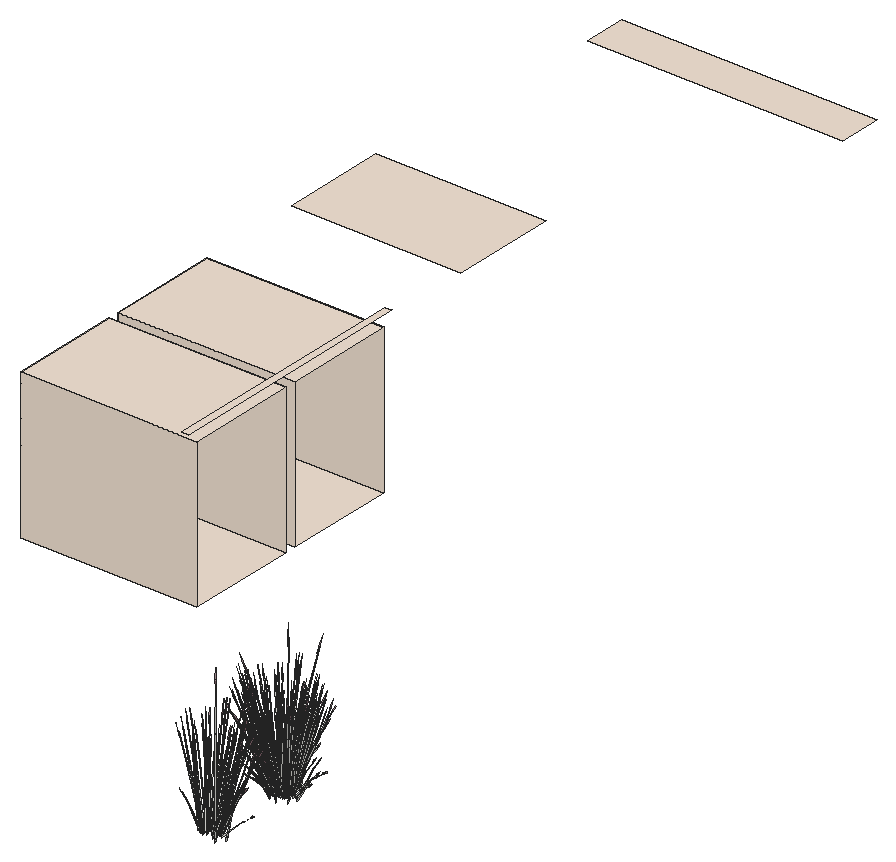
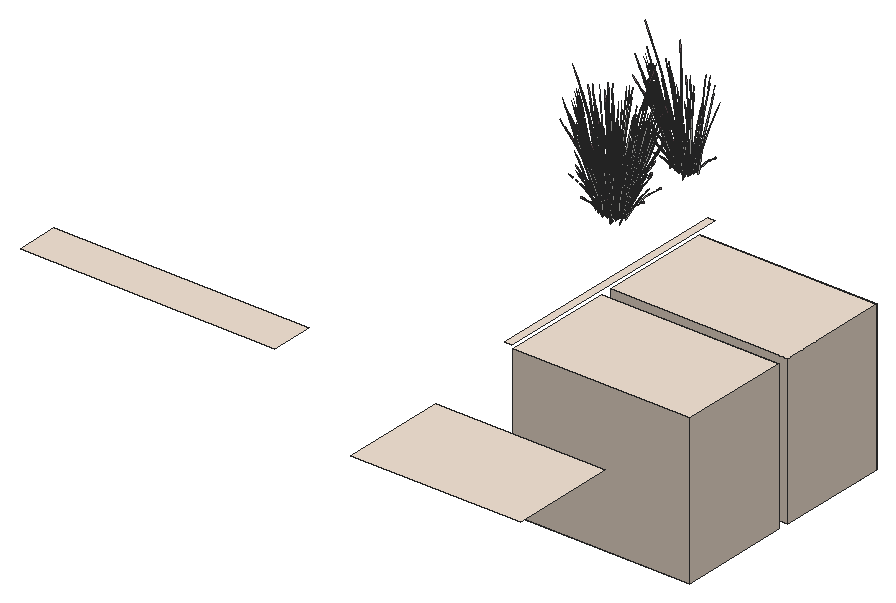
# SketchUp Ruby script. Lengths in inches.
U = 1.inch
M = Sketchup.active_model
def pt(a) = Geom::Point3d.new(a.map { |v| v * U })
def face(e, loops, mat)
  f = e.add_face(loops[0].map { |a| pt(a) })
  loops[1..].each { |l| e.add_face(l.map { |a| pt(a) }).erase! }
  f.material = f.back_material = mat if mat
  f
end
# faces: each face lists its corners as indices into pts; further lists are holes
def faces(e, pts, list, mat = nil) = list.each { |f| face(e, (f[0].is_a?(Array) ? f : [f]).map { |l| l.map { |i| pts[i] } }, mat) }
# xy, xz, yz: faces in a plane at the given z, y or x. An outline is a flat list of corners, or four numbers for a rectangle; further outlines are holes
def ring(l) = l.size == 4 ? [[l[0], l[1]], [l[2], l[1]], [l[2], l[3]], [l[0], l[3]]] : l.each_slice(2).to_a
def flat(e, list, mat, &to3) = list.each { |f| face(e, (f[0].is_a?(Array) ? f : [f]).map { |l| ring(l).map { |u, v| to3.(u, v) } }, mat) }
def xy(e, z, list, mat = nil) = flat(e, list, mat) { |x, y| [x, y, z] }
def xz(e, y, list, mat = nil) = flat(e, list, mat) { |x, z| [x, y, z] }
def yz(e, x, list, mat = nil) = flat(e, list, mat) { |y, z| [x, y, z] }
def lines(e, pts, list) = list.each { |a, b| e.add_line(pt(pts[a]), pt(pts[b])) }
# prism: a flat outline (further loops are holes) pulled along v
def prism(e, loops, v, mat = nil)
  f = face(e, loops, mat); d = Geom::Vector3d.new(v.map { |x| x * U })
  f.pushpull(f.normal.samedirection?(d) ? d.length : -d.length)
end
def box(e, o, s, mat = nil) = prism(e, [[o, [o[0] + s[0], o[1], o[2]], [o[0] + s[0], o[1] + s[1], o[2]], [o[0], o[1] + s[1], o[2]]]], [0, 0, s[2]], mat)
def at(x, y, z, deg = 0) = Geom::Transformation.translation(pt([x, y, z])) * Geom::Transformation.rotation(ORIGIN, Z_AXIS, deg.degrees)
def axes(o, x, y, z) = Geom::Transformation.new([*x, 0, *y, 0, *z, 0, *pt(o).to_a, 1])
def part(name) = M.definitions.add(name)
# library, detail: a bought-in or finely detailed component or shape, given as its bounding box
def library(name, o, s) = part(name).tap { |d| box(d.entities, o, s) }
def detail(e, o, s) = box(e.add_group.entities, o, s)
def put(e, d, t, mat = nil) = e.add_instance(d, t).tap { |i| i.material = mat if mat }
def group(e, t, mat = nil) = e.add_group.tap { |g| g.transformation = t; g.material = mat if mat }.entities
root = M.entities
M.materials.add("C01_Vanilla_Cream").color = [244, 228, 212]
M.materials.add("LightPink_Translucent").color = [144, 107, 117]
M.materials["LightPink_Translucent"].alpha = 0.75
c1 = part("blade")
p = [[2.15,0.21,22],[0,0.17,0],[0.09,0.45,0],[2.18,0.31,22],[2.29,0.31,22],[0.38,0.45,0],
  [2.48,0.24,33],[2.49,0.24,33],[2.48,0.22,33]]
faces(c1.entities,p,[[0,1,2,3],[4,5,2,3],[6,3,4,7],[8,0,3,6]])
c2 = part("seeds")
p = [[0.3,-0.1,1.38],[-0.01,-0.03,1.59],[-0.01,-0.03,0.03],[0.14,-0.07,-0.07],[0.29,-0.03,3],[0.15,0.01,3.11]]
faces(c2.entities,p,[[0,1,2,3],[1,0,4,5]],"LightPink_Translucent")
c3 = part("blade with seeds")
put(c3.entities,c1,at(0,0,0))
put(c3.entities,c2,axes([2.4,0.25,30.99],[1.5799,-0.05474,1.17369],[-0.12525,1.92788,0.29478],[-0.07173,-0.02425,1.56792]))
xy(root,351,[[240,327,290,358.5],[240,361.5,290,393]],"C01_Vanilla_Cream")
xy(root,393,[[240,327,290,358.5],[240,361.5,290,393],[240,423,288,453]],"C01_Vanilla_Cream")
xy(root,396,[[288,324,290,396]],"C01_Vanilla_Cream")
xy(root,432,[[288,468,360,480]],"C01_Vanilla_Cream")
xz(root,327,[[240,351,290,393]],"C01_Vanilla_Cream")
xz(root,358.5,[[240,351,290,393]],"C01_Vanilla_Cream")
xz(root,361.5,[[240,351,290,393]],"C01_Vanilla_Cream")
xz(root,393,[[240,351,290,393]],"C01_Vanilla_Cream")
yz(root,240,[[327,351,358.5,393],[361.5,351,393,393]],"C01_Vanilla_Cream")
put(root,c3,axes([354.47,247.52,351.54],[-0.09091,0.06396,1.31208],[0.00773,0.46734,-0.2075],[-0.20839,0.06078,0.10523]))
put(root,c3,axes([355.07,247.46,351.51],[-0.15083,0.44814,-0.38324],[-0.51712,-0.15361,-0.29685],[-0.2082,0.04109,0.7333]))
put(root,c3,axes([355.05,247.08,351.78],[0.28012,0.44611,-0.0912],[-0.49717,0.21923,-0.50621],[-0.20951,0.05886,0.76918]))
put(root,c3,axes([360.58,249.01,350.95],[-0.10656,-0.41414,-0.02619],[0.50364,-0.09521,-0.11874],[0.10517,0.02626,0.39164]))
put(root,c3,axes([359.27,249,351.78],[0.02981,-0.50103,-0.0912],[0.56442,0.01369,-0.50621],[0.21738,0.0348,0.76918]))
put(root,c3,axes([359.1875,248.8,351.79],[-0.31678,-0.30846,0.2656],[0.36171,-0.29199,-0.3429],[0.18378,0.04443,0.65611]))
put(root,c3,axes([359.76,248.7,351.54],[0.11943,-0.00833,1.31208],[0.32759,-0.38275,-0.2075],[0.21244,0.05052,0.10523]))
put(root,c3,axes([354.99,248.33,351.55],[-0.13808,-0.45342,0.36002],[0.54163,-0.07869,0.29685],[-0.15963,0.10664,0.74497]))
put(root,c3,axes([354.88,248.24,351.55],[-0.3822,-0.20719,0.04823],[0.22252,-0.29505,0.37966],[-0.12254,0.09539,0.57892]))
put(root,c3,axes([355.06,247.69,350.91],[0.19317,-0.10421,1.28532],[0.16263,0.48153,0.10393],[-0.30326,0.10883,0.54946]))
put(root,c3,axes([359.3,248.76,351.74],[0.55654,0.01186,-0.53284],[-0.03738,0.49951,0.0643],[0.23578,0.05271,0.75375]))
put(root,c3,axes([355.32,248.18,351.79],[0.48462,-0.07041,0.2656],[0.12797,0.4025,-0.3429],[-0.13888,0.10811,0.65611]))
put(root,c3,axes([353.46,248,351.53],[0.07105,0.01321,1.33037],[0.2198,0.43529,-0.12571],[-0.14545,0.11425,0.23543]))
put(root,c3,axes([359.64,248.97,351.39],[0.31678,0.30846,-0.2656],[-0.36171,0.29199,0.3429],[0.18378,0.04443,0.65611]))
put(root,c3,axes([359.47,249.08,351.55],[-0.02803,0.37463,0.04823],[-0.42332,-0.01027,0.37966],[0.16216,0.0392,0.57892]))
put(root,c3,axes([354.93,248.41,351.39],[-0.48462,0.07041,-0.2656],[-0.12797,-0.4025,0.3429],[-0.13888,0.10811,0.65611]))
put(root,c3,axes([359.51,248.97,351.55],[-0.41051,0.32462,0.36002],[-0.35404,-0.34474,0.29685],[0.1926,0.05988,0.74497]))
put(root,c3,axes([354.22,249.32,352.23],[0.49129,0.13151,-0.04866],[-0.15113,0.40475,-0.22062],[-0.08035,0.06145,0.72768]))
put(root,c3,axes([358.21,249.34,351.79],[-0.08599,-0.39682,0.2656],[0.49155,-0.10478,-0.3429],[0.13203,0.11372,0.65611]))
put(root,c3,axes([358.5,248.18,350.91],[-0.2068,-0.08488,1.28532],[0.42797,-0.35609,0.10393],[0.26673,0.16064,0.54946]))
put(root,c3,axes([358.54,247.06,351.36],[-0.48108,-0.25598,1.03712],[0.50798,-0.39855,0.44749],[0.15521,0.24018,1.00248]))
put(root,c3,axes([355.07,248.14,351.78],[0.515,0.27165,-0.0912],[-0.2967,0.3934,-0.50621],[-0.1455,0.13675,0.76918]))
put(root,c3,axes([358.16,249.55,351.78],[0.33176,-0.4217,-0.0912],[0.48044,0.24295,-0.50621],[0.16701,0.11914,0.76918]))
put(root,c3,axes([355.76,248.02,350.91],[0.13906,-0.15138,1.28532],[0.35111,0.40859,0.10393],[-0.24082,0.18608,0.54946]))
put(root,c3,axes([355.33,248.46,351.51],[0.14302,0.44985,-0.38324],[-0.54163,0.07869,-0.29685],[-0.15522,0.12083,0.7333]))
put(root,c3,axes([355.98,248.98,351.79],[0.3767,-0.25939,0.2656],[0.3566,0.29618,-0.3429],[-0.05426,0.15048,0.65611]))
put(root,c3,axes([357.73,249.9,351.53],[0.00165,-0.05965,1.33037],[0.47711,-0.26315,-0.12571],[0.16572,0.09393,0.23543]))
put(root,c3,axes([358.5,247.55,350.13],[-0.01521,-0.46386,1.05954],[0.68831,0.12024,0.44862],[-0.1628,0.25382,1.00012]))
put(root,c3,axes([355.63,249.21,351.55],[-0.45752,-0.02296,0.04823],[0.01254,-0.34663,0.37966],[-0.04787,0.13278,0.57892]))
put(root,c3,axes([355.78,249.24,351.55],[-0.39645,-0.33614,0.36002],[0.42102,-0.2899,0.29685],[-0.07313,0.15771,0.74497]))
put(root,c3,axes([358.56,249.34,351.51],[0.54938,-0.11711,-0.38324],[0.0961,0.44351,-0.29685],[0.14756,0.1271,0.7333]))
put(root,c3,axes([357.03,249.4,351.79],[0.16784,-0.37886,0.2656],[0.48968,0.1105,-0.3429],[0.0449,0.15254,0.65611]))
put(root,c3,axes([358.29,249.7,351.55],[-0.25304,0.31296,0.04823],[-0.36033,-0.18221,0.37966],[0.11649,0.10034,0.57892]))
put(root,c3,axes([357.69,250.76,352.23],[0.38473,-0.28263,-0.04866],[0.35252,0.30954,-0.22062],[0.02482,0.08771,0.72768]))
put(root,c3,axes([358.39,249.61,351.55],[-0.55374,0.11306,0.36002],[-0.0961,-0.44351,0.29685],[0.13023,0.13071,0.74497]))
put(root,c3,axes([355.66,248.39,350.91],[0.10366,-0.16934,1.28532],[0.43488,0.35044,0.10393],[-0.19618,0.21841,0.54946]))
put(root,c3,axes([356.88,249.75,351.55],[-0.41024,0.16744,0.04823],[-0.2008,-0.30532,0.37966],[0.03962,0.13459,0.57892]))
put(root,c3,axes([355.78,249.34,351.39],[-0.3767,0.25939,-0.2656],[-0.3566,-0.29618,0.3429],[-0.05426,0.15048,0.65611]))
put(root,c3,axes([354.48,249.27,351.54],[-0.01384,0.09749,1.31208],[0.39274,0.33916,-0.2075],[-0.10282,0.16039,0.10523]))
put(root,c3,axes([355.74,249.05,352.05],[0.61188,0.02441,-0.10123],[-0.01672,0.46217,-0.56189],[-0.0425,0.178,0.85379]))
put(root,c3,axes([356.87,249.5625,351.78],[0.54481,-0.22937,-0.0912],[0.26773,0.4071,-0.50621],[0.07188,0.17155,0.76918]))
put(root,c3,axes([357.03,249.71,351.8],[-0.54859,-0.1288,0.39962],[0.18759,-0.42344,0.32951],[0.03297,0.16652,0.82692]))
put(root,c3,axes([356.02,250.35,350.07],[-0.01441,-0.29294,0.86145],[0.36003,0.20894,0.63294],[-0.07081,0.13963,0.18974]))
put(root,c3,axes([356.15,249.22,351.75],[0.39855,0.33102,-0.4254],[-0.42102,0.2899,-0.32951],[-0.06064,0.16819,0.81396]))
put(root,c3,axes([357.34,249.54,351.51],[0.54728,0.1235,-0.38324],[-0.18759,0.42344,-0.29685],[0.05018,0.17048,0.7333]))
put(root,c3,axes([357.65,248.67,350.91],[-0.12726,-0.15818,1.28532],[0.58807,-0.13317,0.10393],[0.13291,0.24832,0.54946]))
put(root,c3,axes([357.09,249.8,351.39],[-0.16784,0.37886,-0.2656],[-0.48968,-0.1105,0.3429],[0.0449,0.15254,0.65611]))
put(root,c3,axes([356.03,249.07,352],[-0.01449,0.45571,-0.59145],[-0.61002,-0.03061,0.07138],[-0.06438,0.19306,0.83667]))
put(root,c3,axes([354.4375,250.27,351.53],[0.06316,-0.02974,1.33037],[0.52204,0.19785,-0.12571],[-0.01227,0.16473,0.23543]))
put(root,c3,axes([356.61,248.75,350.91],[-0.01363,-0.18909,1.28532],[0.5906,0.12544,0.10393],[-0.03653,0.26947,0.54946]))
put(root,c3,axes([357.14,249.46,351.74],[0.26572,0.40059,-0.53284],[-0.54698,0.22325,0.0643],[0.06214,0.19355,0.75375]))
put(root,c3,axes([356.74,250.47,351.54],[0.07057,0.07933,1.31208],[0.56952,0.03117,-0.2075],[0.05727,0.17496,0.10523]))
put(root,c3,axes([355.83,249.71,350.52],[0.01223,-0.25433,1.15759],[0.55017,0.13434,0.15997],[-0.04767,0.27105,0.54661]))
put(root,c3,axes([356.25,271.21,350.91],[0.12726,0.15818,1.28532],[-0.58807,0.13317,0.10393],[-0.13291,-0.24832,0.54946]))
put(root,c3,axes([357.22,270.16,351.54],[-0.08515,-0.06907,1.31208],[-0.56828,0.04379,-0.2075],[-0.0907,-0.16522,0.10523]))
put(root,c3,axes([357.82,271.33,351.74],[-0.26572,-0.40059,-0.53284],[0.54698,-0.22325,0.0643],[-0.06214,-0.19355,0.75375]))
put(root,c3,axes([358.92,271.72,351.74],[0.01449,-0.45571,-0.53284],[0.61002,0.03061,0.0643],[0.06438,-0.19306,0.75375]))
put(root,c3,axes([359.77,271.01,351.54],[-0.00537,-0.09805,1.31208],[-0.45391,-0.28338,-0.2075],[0.07018,-0.17178,0.10523]))
put(root,c3,axes([357.87,270.99,351.39],[0.16784,-0.37886,-0.2656],[0.48968,0.1105,0.3429],[-0.0449,-0.15254,0.65611]))
put(root,c3,axes([358.24,271.49,350.91],[-0.10366,0.16934,1.28532],[-0.43488,-0.35044,0.10393],[0.19618,-0.21841,0.54946]))
put(root,c3,axes([359.65,270.66,351.53],[-0.05654,0.03763,1.33037],[-0.55396,-0.12696,-0.12571],[-0.02005,-0.16422,0.23543]))
put(root,c3,axes([357.62,271.25,351.51],[-0.54728,-0.1235,-0.38324],[0.18759,-0.42344,-0.29685],[-0.05018,-0.17048,0.7333]))
put(root,c3,axes([357.95,270.1875,350.07],[0.07142,0.28728,0.86145],[-0.3962,-0.15911,0.63294],[0.04263,-0.1471,0.18974]))
put(root,c3,axes([358.8,271.57,351.51],[-0.39855,-0.33102,-0.38324],[0.42102,-0.2899,-0.29685],[0.06064,-0.16819,0.7333]))
put(root,c3,axes([356.64,269.9375,351.53],[-0.01039,0.05905,1.33037],[-0.51226,0.21431,-0.12571],[-0.15074,-0.10955,0.23543]))
put(root,c3,axes([356.52,270.98,351.82],[0.62019,-0.12663,0.40322],[0.10763,0.49673,0.33247],[-0.14586,-0.1464,0.83437]))
put(root,c3,axes([357.93,271.08,351.55],[0.54859,0.1288,0.36002],[-0.18759,0.42344,0.29685],[-0.03297,-0.16652,0.74497]))
put(root,c3,axes([358.08,271.23,351.78],[-0.54481,0.22937,-0.0912],[-0.26773,-0.4071,-0.50621],[-0.07188,-0.17155,0.76918]))
put(root,c3,axes([359.22,271.74,351.78],[-0.61188,-0.02441,-0.0912],[0.01672,-0.46217,-0.50621],[0.0425,-0.178,0.76918]))
put(root,c3,axes([359.17,271.45,351.39],[0.3767,-0.25939,-0.2656],[0.3566,0.29618,0.3429],[0.05426,-0.15048,0.65611]))
put(root,c3,axes([355.92,270.53,350.07],[0.29042,0.17147,0.86145],[-0.42295,0.10307,0.63294],[-0.0905,-0.13178,0.18974]))
put(root,c3,axes([358.07,271.04,351.55],[0.41024,-0.16744,0.04823],[0.2008,0.30532,0.37966],[-0.03962,-0.13459,0.57892]))
put(root,c3,axes([356.62,271.44,351.74],[-0.47473,-0.23813,-0.53284],[0.33738,-0.41728,0.0643],[-0.172,-0.14218,0.75375]))
put(root,c3,axes([356.45,271.13,351.39],[-0.08599,-0.39682,-0.2656],[0.49155,-0.10478,0.3429],[-0.13203,-0.11372,0.65611]))
put(root,c3,axes([356.67,271.09,351.55],[0.25304,-0.31296,0.04823],[0.36033,0.18221,0.37966],[-0.11649,-0.10034,0.57892]))
put(root,c3,axes([355.4,271.7,350.91],[0.2068,0.08488,1.28532],[-0.42797,0.35609,0.10393],[-0.26673,-0.16064,0.54946]))
put(root,c3,axes([357.92,271.39,351.79],[-0.16784,0.37886,0.2656],[-0.48968,-0.1105,-0.3429],[-0.0449,-0.15254,0.65611]))
put(root,c3,axes([356.4,271.45,351.51],[-0.54938,0.11711,-0.38324],[-0.0961,-0.44351,-0.29685],[-0.14756,-0.1271,0.7333]))
put(root,c3,axes([359.17,271.55,351.55],[0.39645,0.33614,0.36002],[-0.42102,0.2899,0.29685],[0.07313,-0.15771,0.74497]))
put(root,c3,axes([356.78,271.06,352.07],[-0.37157,0.4723,-0.10215],[-0.5381,-0.2721,-0.56695],[-0.18705,-0.13344,0.86148]))
put(root,c3,axes([359.32,271.58,351.55],[0.45752,0.02296,0.04823],[-0.01254,0.34663,0.37966],[0.04787,-0.13278,0.57892]))
put(root,c3,axes([358.98,271.8125,351.79],[-0.3767,0.25939,0.2656],[-0.3566,-0.29618,-0.3429],[0.05426,-0.15048,0.65611]))
put(root,c3,axes([359.64,272.51,351.74],[0.29081,-0.38873,-0.53284],[0.5096,0.27626,0.0643],[0.17364,-0.14084,0.75375]))
put(root,c3,axes([359.625,272.33,351.51],[-0.14302,-0.44985,-0.38324],[0.54163,-0.07869,-0.29685],[0.15522,-0.12083,0.7333]))
put(root,c3,axes([355.36,270.92,351.54],[-0.11979,-0.00348,1.31208],[-0.38137,0.34775,-0.2075],[-0.20349,-0.07106,0.10523]))
put(root,c3,axes([359.88,272.65,351.78],[-0.515,-0.27165,-0.0912],[0.2967,-0.3934,-0.50621],[0.1455,-0.13675,0.76918]))
put(root,c3,axes([357.75,274.14,350.49],[0.48111,0.19866,1.13446],[-0.47133,0.42798,0.44862],[-0.21112,-0.25366,0.95105]))
put(root,c3,axes([356.75,271.45,351.79],[0.08599,0.39682,0.2656],[-0.49155,0.10478,-0.3429],[-0.13203,-0.11372,0.65611]))
put(root,c3,axes([355.27,271.71,351.82],[0.45978,-0.36358,0.40322],[0.39653,0.38611,0.33247],[-0.21571,-0.06707,0.83437]))
put(root,c3,axes([361.15,272.54,351.53],[-0.07272,-0.00374,1.33037],[-0.30197,-0.40092,-0.12571],[0.12127,-0.13182,0.23543]))
put(root,c3,axes([360.29,271.4375,350.07],[-0.18544,0.25079,0.86145],[-0.15939,-0.33694,0.63294],[0.15316,-0.08443,0.18974]))
put(root,c3,axes([360.03,272.38,351.39],[0.48462,-0.07041,-0.2656],[0.12797,0.4025,0.3429],[0.13888,-0.10811,0.65611]))
put(root,c3,axes([355.48,271.71,351.55],[0.02803,-0.37463,0.04823],[0.42332,0.01027,0.37966],[-0.16216,-0.0392,0.57892]))
put(root,c3,axes([355.32,271.83,351.39],[-0.31678,-0.30846,-0.2656],[0.36171,-0.29199,0.3429],[-0.18378,-0.04443,0.65611]))
put(root,c3,axes([359.63,272.62,351.79],[-0.48462,0.07041,0.2656],[-0.12797,-0.4025,-0.3429],[0.13888,-0.10811,0.65611]))
put(root,c3,axes([355.65,272.03,351.74],[-0.55654,-0.01186,-0.53284],[0.03738,-0.49951,0.0643],[-0.23578,-0.05271,0.75375]))
put(root,c3,axes([360.07,272.55,351.55],[0.3822,0.20719,0.04823],[-0.22252,0.29505,0.37966],[0.12254,-0.09539,0.57892]))
put(root,c3,axes([359.96,272.47,351.55],[0.13808,0.45342,0.36002],[-0.54163,0.07869,0.29685],[0.15963,-0.10664,0.74497]))
put(root,c3,axes([361.42,273.01,351.54],[0.07726,-0.07504,1.31208],[-0.09888,-0.46032,-0.2075],[0.19384,-0.08728,0.10523]))
put(root,c3,axes([354.9,271.22,351.53],[0.04127,0.04917,1.33037],[-0.19898,0.44196,-0.12571],[-0.20151,0.0032,0.23543]))
put(root,c3,axes([355.47,272.13,351.51],[-0.40426,0.32635,-0.38324],[-0.35404,-0.34474,-0.29685],[-0.2054,-0.04965,0.7333]))
put(root,c3,axes([355.77,271.99,351.79],[0.31678,0.30846,0.2656],[-0.36171,0.29199,-0.3429],[-0.18378,-0.04443,0.65611]))
put(root,c3,axes([354.56,272.56,350.07],[0.35544,-0.03525,0.86145],[-0.22547,0.31061,0.63294],[-0.17565,-0.04659,0.18974]))
put(root,c3,axes([355.68,271.79,351.78],[-0.02981,0.50103,-0.0912],[-0.56442,-0.01369,-0.50621],[-0.21738,-0.0348,0.76918]))
put(root,c3,axes([359.9,273.71,351.78],[-0.28012,-0.44611,-0.0912],[0.49717,-0.21923,-0.50621],[0.20951,-0.05886,0.76918]))
put(root,c3,axes([359.88,273.33,351.51],[0.15083,-0.44814,-0.38324],[0.51712,0.15361,-0.29685],[0.2082,-0.04109,0.7333]))
put(root,c3,axes([354.96,272.48,350.91],[0.23093,-0.01116,1.28532],[-0.15319,0.4836,0.10393],[-0.32909,-0.02991,0.54946]))
put(root,c3,axes([359.78,273.49,351.74],[0.48922,-0.21758,-0.53284],[0.27264,0.44789,0.0643],[0.23638,-0.05088,0.75375]))
put(root,c3,axes([359.71,273.58,351.79],[-0.46269,-0.13744,0.2656],[0.13495,-0.40096,-0.3429],[0.18628,-0.03677,0.65611]))
put(root,c3,axes([354.86,272.85,351.55],[0.15729,-0.44921,0.36002],[0.51712,0.15361,0.29685],[-0.20336,0.027,0.74497]))
put(root,c3,axes([354.83,272.73,351.55],[-0.20448,-0.33592,0.04823],[0.37288,-0.16442,0.37966],[-0.16437,0.03244,0.57892]))
put(root,c3,axes([360.2,273.53,351.39],[0.46269,0.13744,-0.2656],[-0.13495,0.40096,0.3429],[0.18628,-0.03677,0.65611]))
put(root,c3,axes([354.76,272.9,351.39],[-0.46269,-0.13744,-0.2656],[0.13495,-0.40096,0.3429],[-0.18628,0.03677,0.65611]))
put(root,c3,axes([358.93,273.04,350.91],[-0.23093,0.01116,1.28532],[0.15319,-0.4836,0.10393],[0.32909,0.02991,0.54946]))
put(root,c3,axes([360.13,273.7,351.55],[0.20448,0.33592,0.04823],[-0.37288,0.16442,0.37966],[0.16437,-0.03244,0.57892]))
put(root,c3,axes([360.09,273.58,351.55],[-0.15729,0.44921,0.36002],[-0.51712,-0.15361,0.29685],[0.20336,-0.027,0.74497]))
put(root,c3,axes([355.24,272.85,351.79],[0.46269,0.13744,0.2656],[-0.13495,0.40096,-0.3429],[-0.18628,0.03677,0.65611]))
put(root,c3,axes([356.17,272.83,350.51],[0.15825,-0.07127,1.32798],[0.05457,0.4976,0.10393],[-0.34278,0.06603,0.47463]))
put(root,c3,axes([361.18,273.62,350.07],[-0.34399,0.08133,0.86145],[0.16192,-0.33614,0.63294],[0.18249,0.023,0.18974]))
put(root,c3,axes([361.02,275.04,351.53],[-0.05034,-0.04313,1.33037],[0.11012,-0.46232,-0.12571],[0.1983,-0.02954,0.23543]))
put(root,c3,axes([354.47,273.16,351.54],[-0.09091,0.06396,1.31208],[0.00773,0.46734,-0.2075],[-0.20839,0.06078,0.10523]))
put(root,c3,axes([355.07,273.1,351.51],[-0.15083,0.44814,-0.38324],[-0.51712,-0.15361,-0.29685],[-0.2082,0.04109,0.7333]))
put(root,c3,axes([355.05,272.72,351.78],[0.28012,0.44611,-0.0912],[-0.49717,0.21923,-0.50621],[-0.20951,0.05886,0.76918]))
put(root,c3,axes([360.58,274.65,350.95],[-0.10656,-0.41414,-0.02619],[0.50364,-0.09521,-0.11874],[0.10517,0.02626,0.39164]))
put(root,c3,axes([359.27,274.64,351.78],[0.02981,-0.50103,-0.0912],[0.56442,0.01369,-0.50621],[0.21738,0.0348,0.76918]))
put(root,c3,axes([359.1875,274.44,351.79],[-0.31678,-0.30846,0.2656],[0.36171,-0.29199,-0.3429],[0.18378,0.04443,0.65611]))
put(root,c3,axes([359.76,274.34,351.54],[0.11943,-0.00833,1.31208],[0.32759,-0.38275,-0.2075],[0.21244,0.05052,0.10523]))
put(root,c3,axes([354.99,273.97,351.55],[-0.13808,-0.45342,0.36002],[0.54163,-0.07869,0.29685],[-0.15963,0.10664,0.74497]))
put(root,c3,axes([354.88,273.88,351.55],[-0.3822,-0.20719,0.04823],[0.22252,-0.29505,0.37966],[-0.12254,0.09539,0.57892]))
put(root,c3,axes([355.06,273.33,350.91],[0.19317,-0.10421,1.28532],[0.16263,0.48153,0.10393],[-0.30326,0.10883,0.54946]))
put(root,c3,axes([359.3,274.4,351.74],[0.55654,0.01186,-0.53284],[-0.03738,0.49951,0.0643],[0.23578,0.05271,0.75375]))
put(root,c3,axes([355.32,273.8125,351.79],[0.48462,-0.07041,0.2656],[0.12797,0.4025,-0.3429],[-0.13888,0.10811,0.65611]))
put(root,c3,axes([353.46,273.64,351.53],[0.07105,0.01321,1.33037],[0.2198,0.43529,-0.12571],[-0.14545,0.11425,0.23543]))
put(root,c3,axes([354.05,275.02,350.07],[0.23202,-0.22328,0.86145],[0.09155,0.35348,0.63294],[-0.16768,0.06329,0.18974]))
put(root,c3,axes([359.64,274.61,351.39],[0.31678,0.30846,-0.2656],[-0.36171,0.29199,0.3429],[0.18378,0.04443,0.65611]))
put(root,c3,axes([359.47,274.72,351.55],[-0.02803,0.37463,0.04823],[-0.42332,-0.01027,0.37966],[0.16216,0.0392,0.57892]))
put(root,c3,axes([354.93,274.05,351.39],[-0.48462,0.07041,-0.2656],[-0.12797,-0.4025,0.3429],[-0.13888,0.10811,0.65611]))
put(root,c3,axes([359.51,274.6,351.55],[-0.41051,0.32462,0.36002],[-0.35404,-0.34474,0.29685],[0.1926,0.05988,0.74497]))
put(root,c3,axes([354.22,274.96,352.23],[0.49129,0.13151,-0.04866],[-0.15113,0.40475,-0.22062],[-0.08035,0.06145,0.72768]))
put(root,c3,axes([358.21,274.98,351.79],[-0.08599,-0.39682,0.2656],[0.49155,-0.10478,-0.3429],[0.13203,0.11372,0.65611]))
put(root,c3,axes([358.5,273.8125,350.91],[-0.2068,-0.08488,1.28532],[0.42797,-0.35609,0.10393],[0.26673,0.16064,0.54946]))
put(root,c3,axes([358.54,272.7,351.36],[-0.48108,-0.25598,1.03712],[0.50798,-0.39855,0.44749],[0.15521,0.24018,1.00248]))
put(root,c3,axes([355.07,273.78,351.78],[0.515,0.27165,-0.0912],[-0.2967,0.3934,-0.50621],[-0.1455,0.13675,0.76918]))
put(root,c3,axes([359.26,274.78,350.07],[-0.31347,-0.14166,0.86145],[0.40476,-0.14393,0.63294],[0.10917,0.12192,0.18974]))
put(root,c3,axes([358.16,275.19,351.78],[0.33176,-0.4217,-0.0912],[0.48044,0.24295,-0.50621],[0.16701,0.11914,0.76918]))
put(root,c3,axes([355.76,273.66,350.91],[0.13906,-0.15138,1.28532],[0.35111,0.40859,0.10393],[-0.24082,0.18608,0.54946]))
put(root,c3,axes([355.33,274.1,351.51],[0.14302,0.44985,-0.38324],[-0.54163,0.07869,-0.29685],[-0.15522,0.12083,0.7333]))
put(root,c3,axes([355.98,274.62,351.79],[0.3767,-0.25939,0.2656],[0.3566,0.29618,-0.3429],[-0.05426,0.15048,0.65611]))
put(root,c3,axes([357.73,275.54,351.53],[0.00165,-0.05965,1.33037],[0.47711,-0.26315,-0.12571],[0.16572,0.09393,0.23543]))
put(root,c3,axes([358.5,273.1875,350.13],[-0.01521,-0.46386,1.05954],[0.68831,0.12024,0.44862],[-0.1628,0.25382,1.00012]))
put(root,c3,axes([355.63,274.85,351.55],[-0.45752,-0.02296,0.04823],[0.01254,-0.34663,0.37966],[-0.04787,0.13278,0.57892]))
put(root,c3,axes([355.78,274.88,351.55],[-0.39645,-0.33614,0.36002],[0.42102,-0.2899,0.29685],[-0.07313,0.15771,0.74497]))
put(root,c3,axes([358.56,274.98,351.51],[0.54938,-0.11711,-0.38324],[0.0961,0.44351,-0.29685],[0.14756,0.1271,0.7333]))
put(root,c3,axes([357.03,275.04,351.79],[0.16784,-0.37886,0.2656],[0.48968,0.1105,-0.3429],[0.0449,0.15254,0.65611]))
put(root,c3,axes([358.29,275.34,351.55],[-0.25304,0.31296,0.04823],[-0.36033,-0.18221,0.37966],[0.11649,0.10034,0.57892]))
put(root,c3,axes([357.69,276.39,352.23],[0.38473,-0.28263,-0.04866],[0.35252,0.30954,-0.22062],[0.02482,0.08771,0.72768]))
put(root,c3,axes([358.39,275.25,351.55],[-0.55374,0.11306,0.36002],[-0.0961,-0.44351,0.29685],[0.13023,0.13071,0.74497]))
put(root,c3,axes([355.66,274.03,350.91],[0.10366,-0.16934,1.28532],[0.43488,0.35044,0.10393],[-0.19618,0.21841,0.54946]))
put(root,c3,axes([356.88,275.39,351.55],[-0.41024,0.16744,0.04823],[-0.2008,-0.30532,0.37966],[0.03962,0.13459,0.57892]))
put(root,c3,axes([355.78,274.98,351.39],[-0.3767,0.25939,-0.2656],[-0.3566,-0.29618,0.3429],[-0.05426,0.15048,0.65611]))
put(root,c3,axes([354.48,274.91,351.54],[-0.01384,0.09749,1.31208],[0.39274,0.33916,-0.2075],[-0.10282,0.16039,0.10523]))
put(root,c3,axes([355.74,274.6875,352.05],[0.61188,0.02441,-0.10123],[-0.01672,0.46217,-0.56189],[-0.0425,0.178,0.85379]))
put(root,c3,axes([356.87,275.2,351.78],[0.54481,-0.22937,-0.0912],[0.26773,0.4071,-0.50621],[0.07188,0.17155,0.76918]))
put(root,c3,axes([357.03,275.35,351.8],[-0.54859,-0.1288,0.39962],[0.18759,-0.42344,0.32951],[0.03297,0.16652,0.82692]))
put(root,c3,axes([356.02,275.99,350.07],[-0.01441,-0.29294,0.86145],[0.36003,0.20894,0.63294],[-0.07081,0.13963,0.18974]))
put(root,c3,axes([356.15,274.86,351.75],[0.39855,0.33102,-0.4254],[-0.42102,0.2899,-0.32951],[-0.06064,0.16819,0.81396]))
put(root,c3,axes([357.34,275.18,351.51],[0.54728,0.1235,-0.38324],[-0.18759,0.42344,-0.29685],[0.05018,0.17048,0.7333]))
put(root,c3,axes([357.65,274.31,350.91],[-0.12726,-0.15818,1.28532],[0.58807,-0.13317,0.10393],[0.13291,0.24832,0.54946]))
put(root,c3,axes([357.09,275.44,351.39],[-0.16784,0.37886,-0.2656],[-0.48968,-0.1105,0.3429],[0.0449,0.15254,0.65611]))
put(root,c3,axes([356.03,274.71,352],[-0.01449,0.45571,-0.59145],[-0.61002,-0.03061,0.07138],[-0.06438,0.19306,0.83667]))
put(root,c3,axes([354.4375,275.91,351.53],[0.06316,-0.02974,1.33037],[0.52204,0.19785,-0.12571],[-0.01227,0.16473,0.23543]))
put(root,c3,axes([356.61,274.39,350.91],[-0.01363,-0.18909,1.28532],[0.5906,0.12544,0.10393],[-0.03653,0.26947,0.54946]))
put(root,c3,axes([357.14,275.1,351.74],[0.26572,0.40059,-0.53284],[-0.54698,0.22325,0.0643],[0.06214,0.19355,0.75375]))
put(root,c3,axes([356.74,276.11,351.54],[0.07057,0.07933,1.31208],[0.56952,0.03117,-0.2075],[0.05727,0.17496,0.10523]))
put(root,c3,axes([355.83,275.35,350.52],[0.01223,-0.25433,1.15759],[0.55017,0.13434,0.15997],[-0.04767,0.27105,0.54661]))
